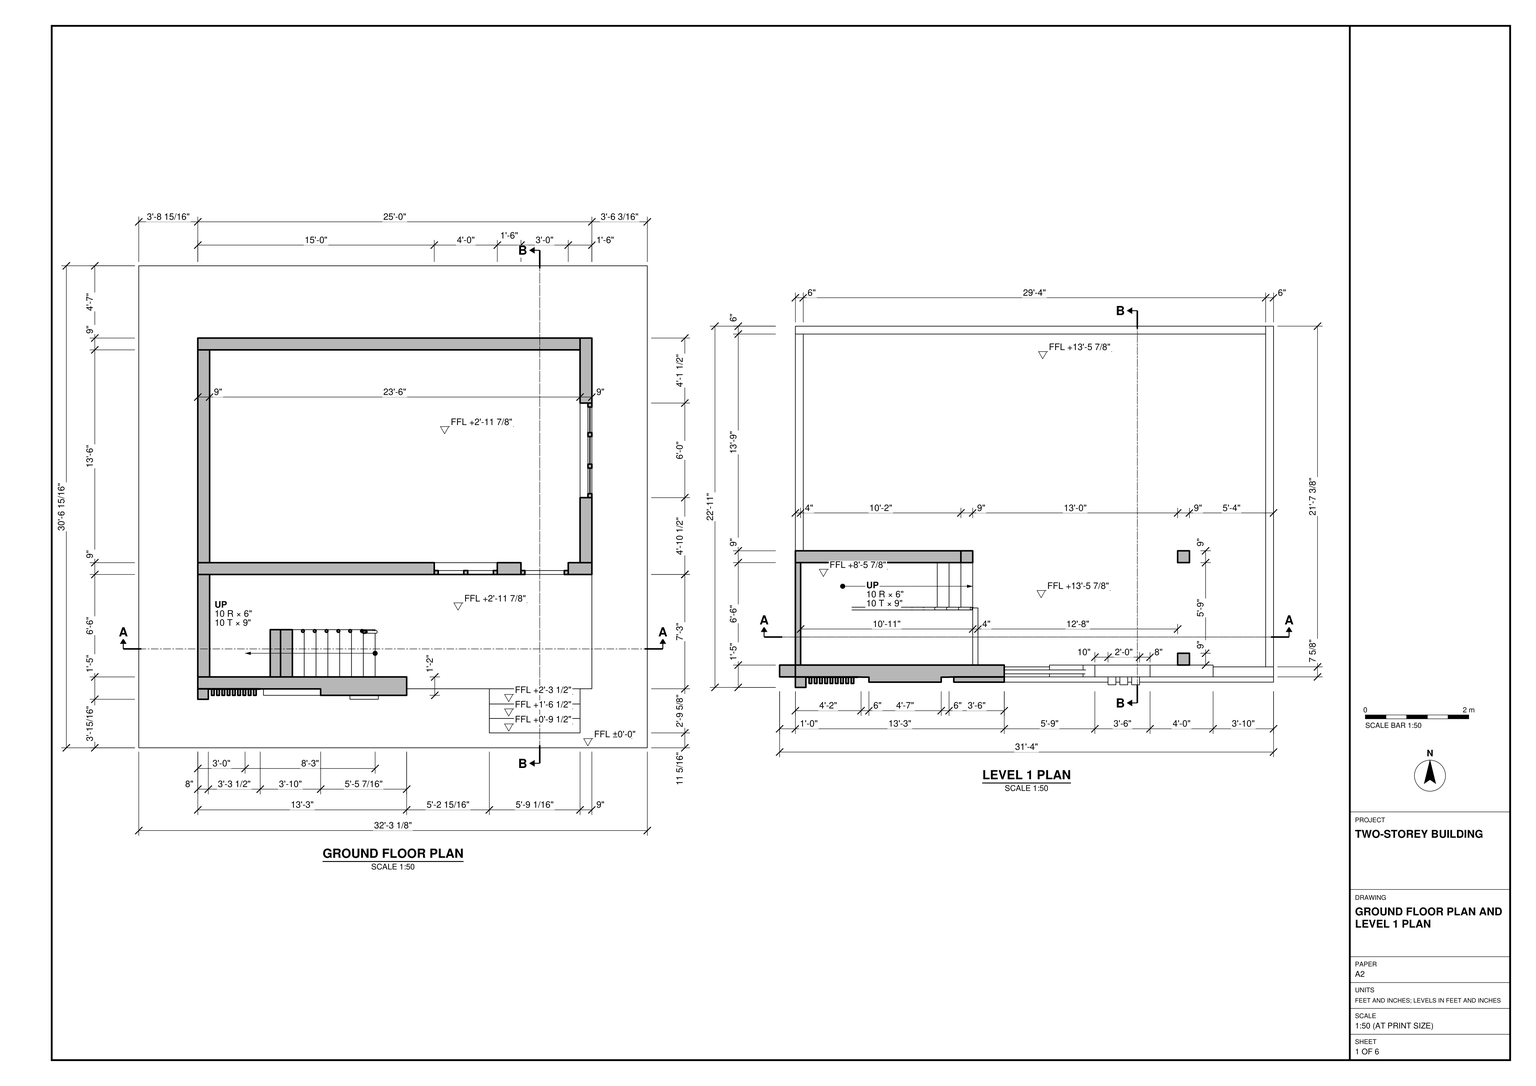
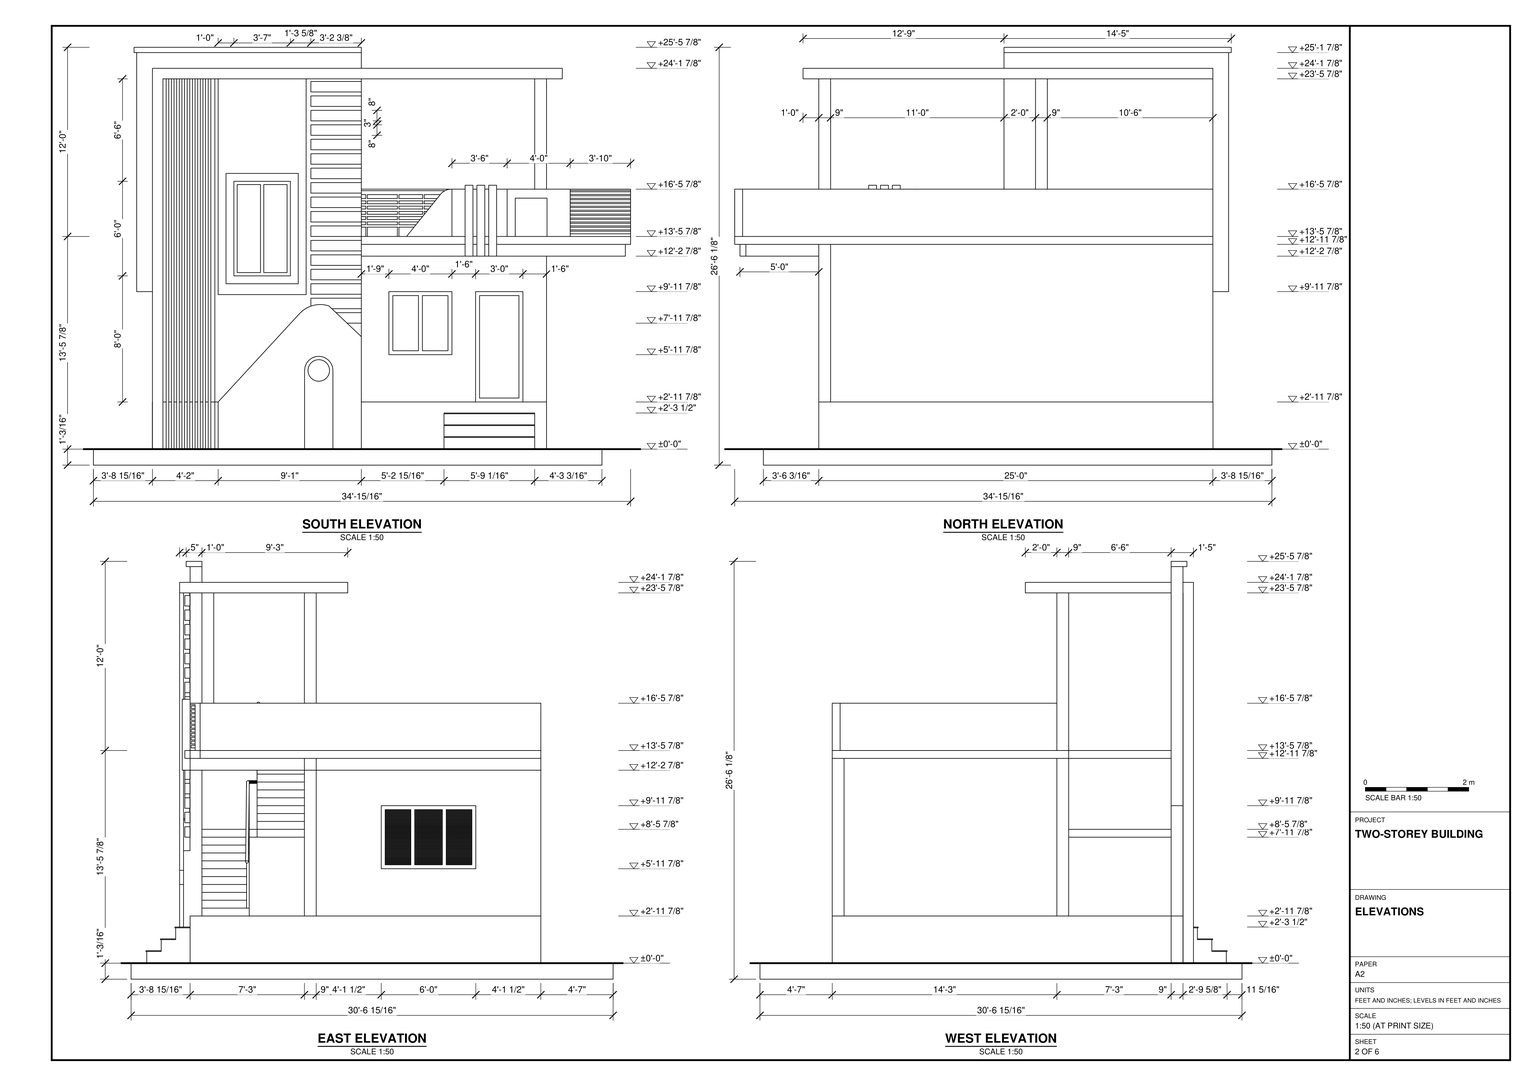
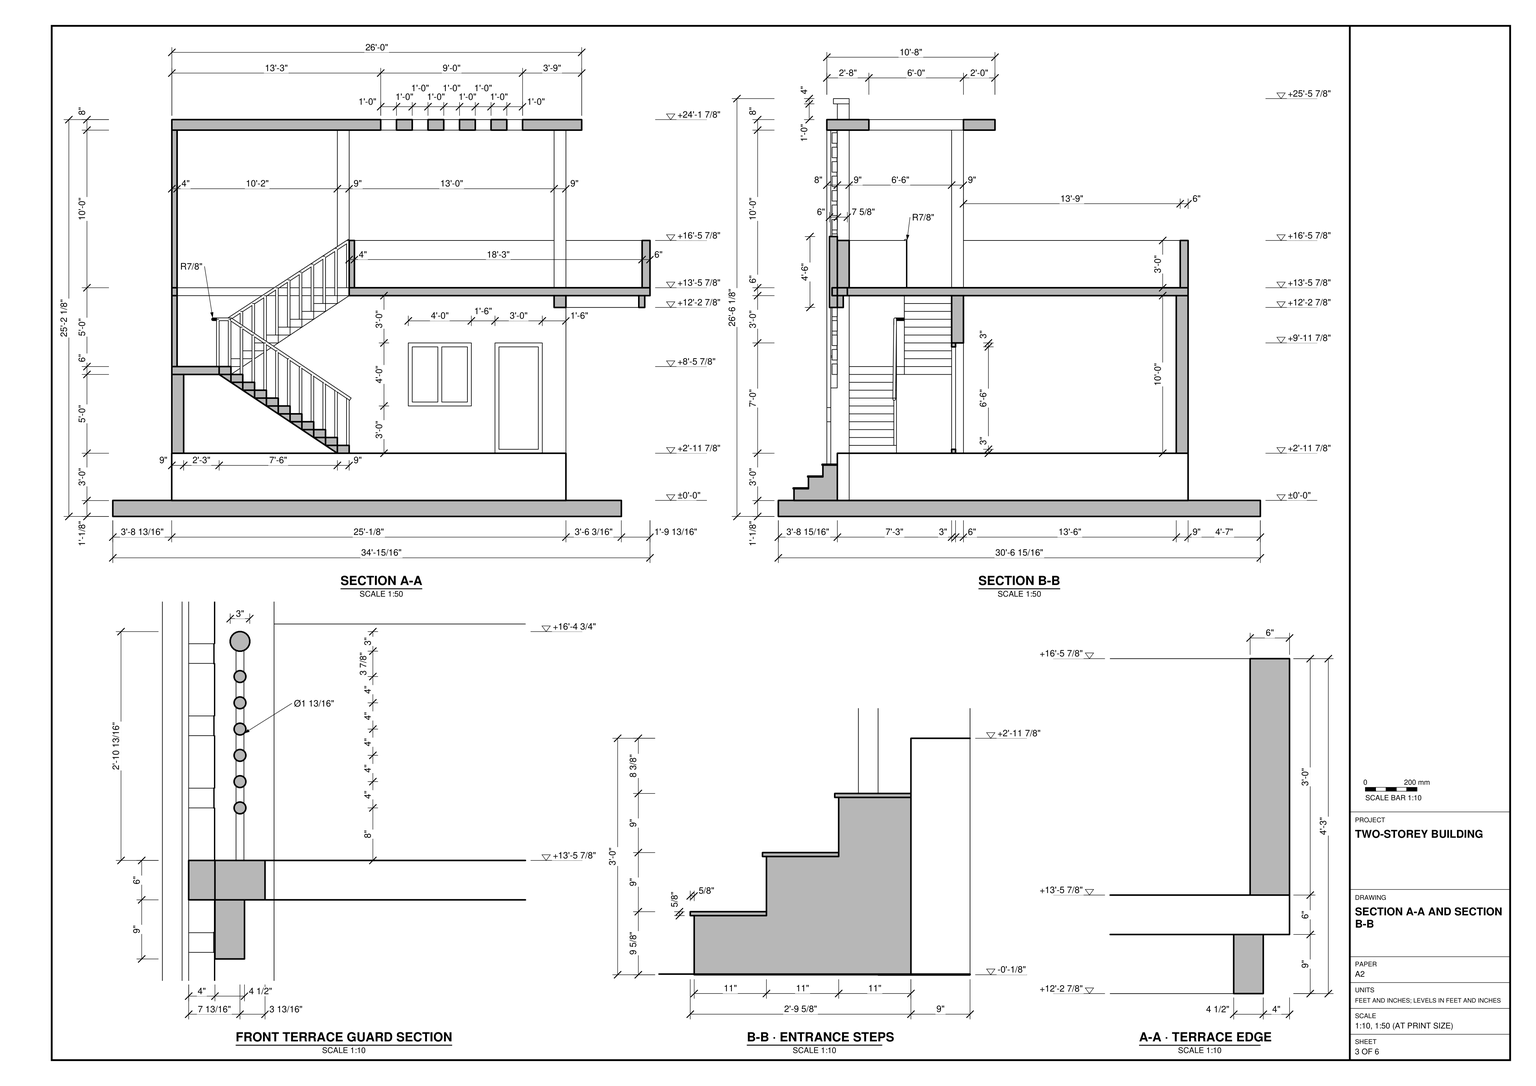
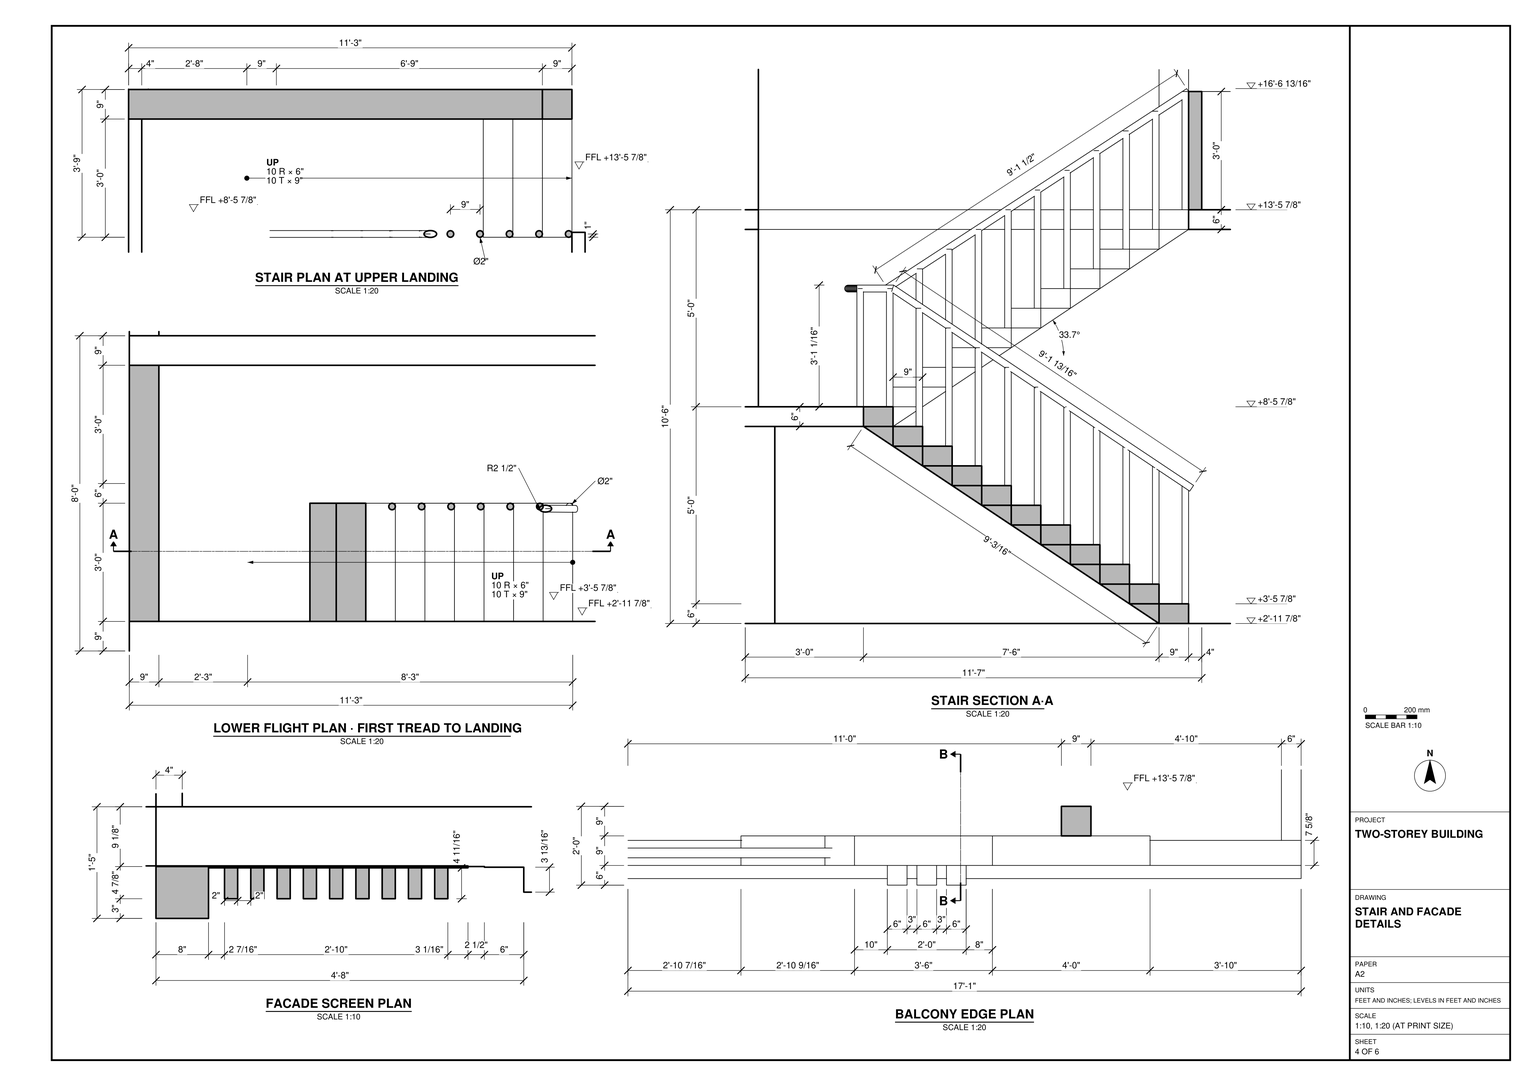
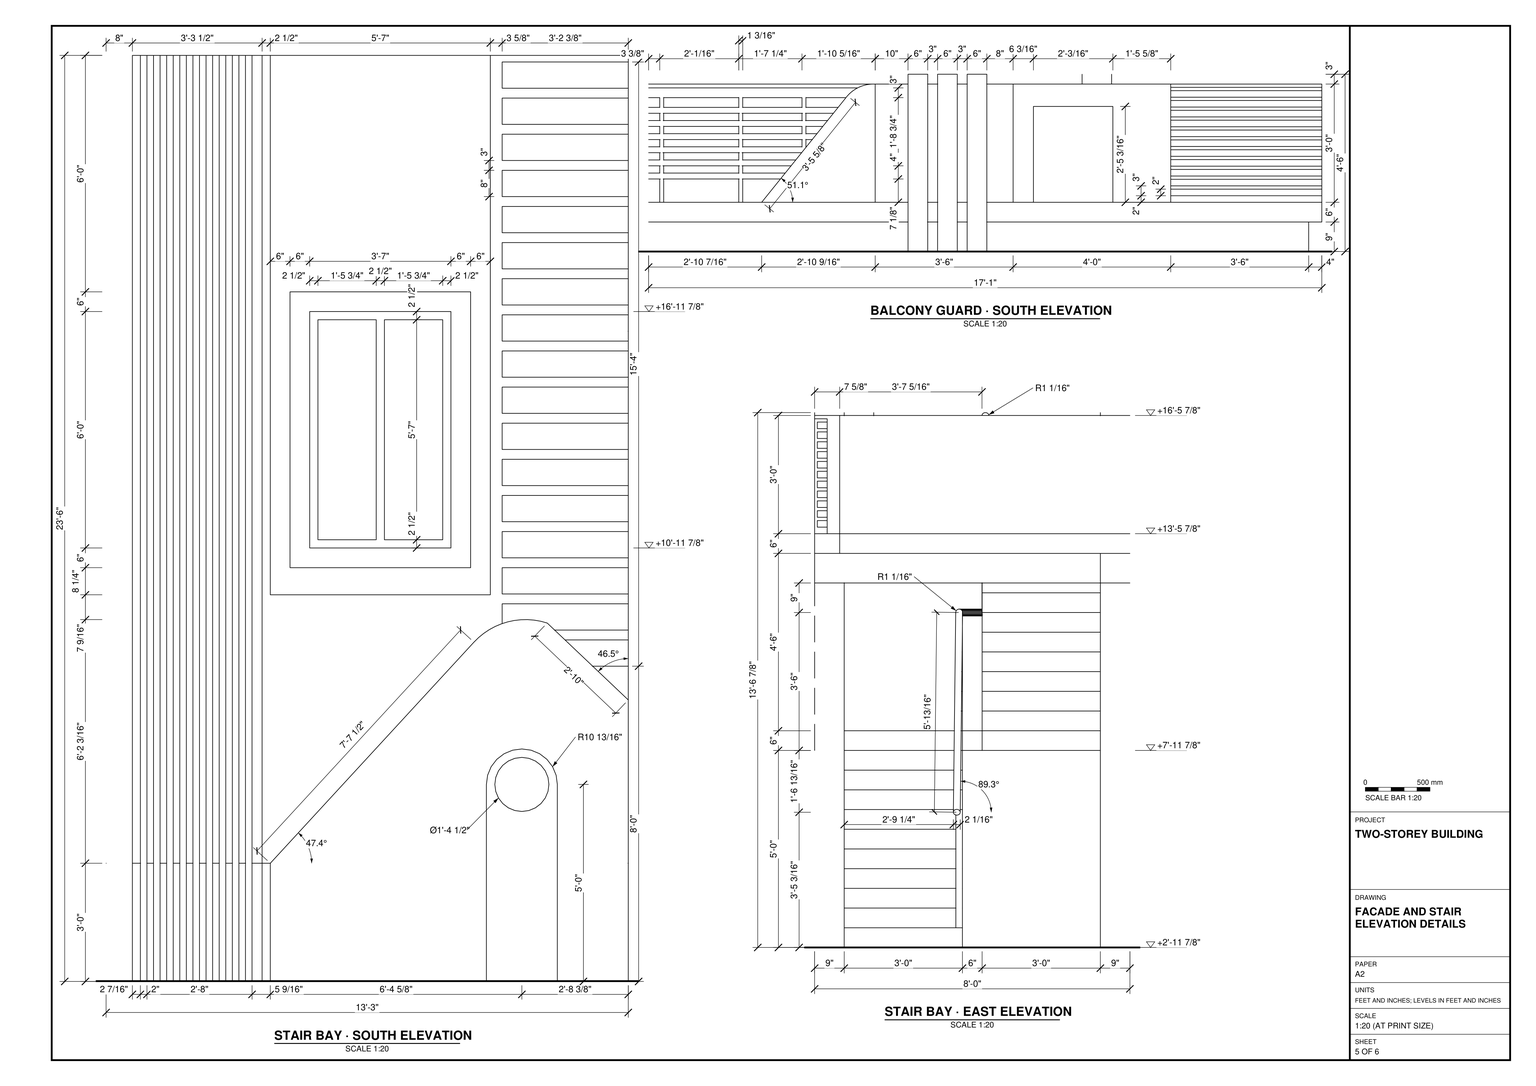
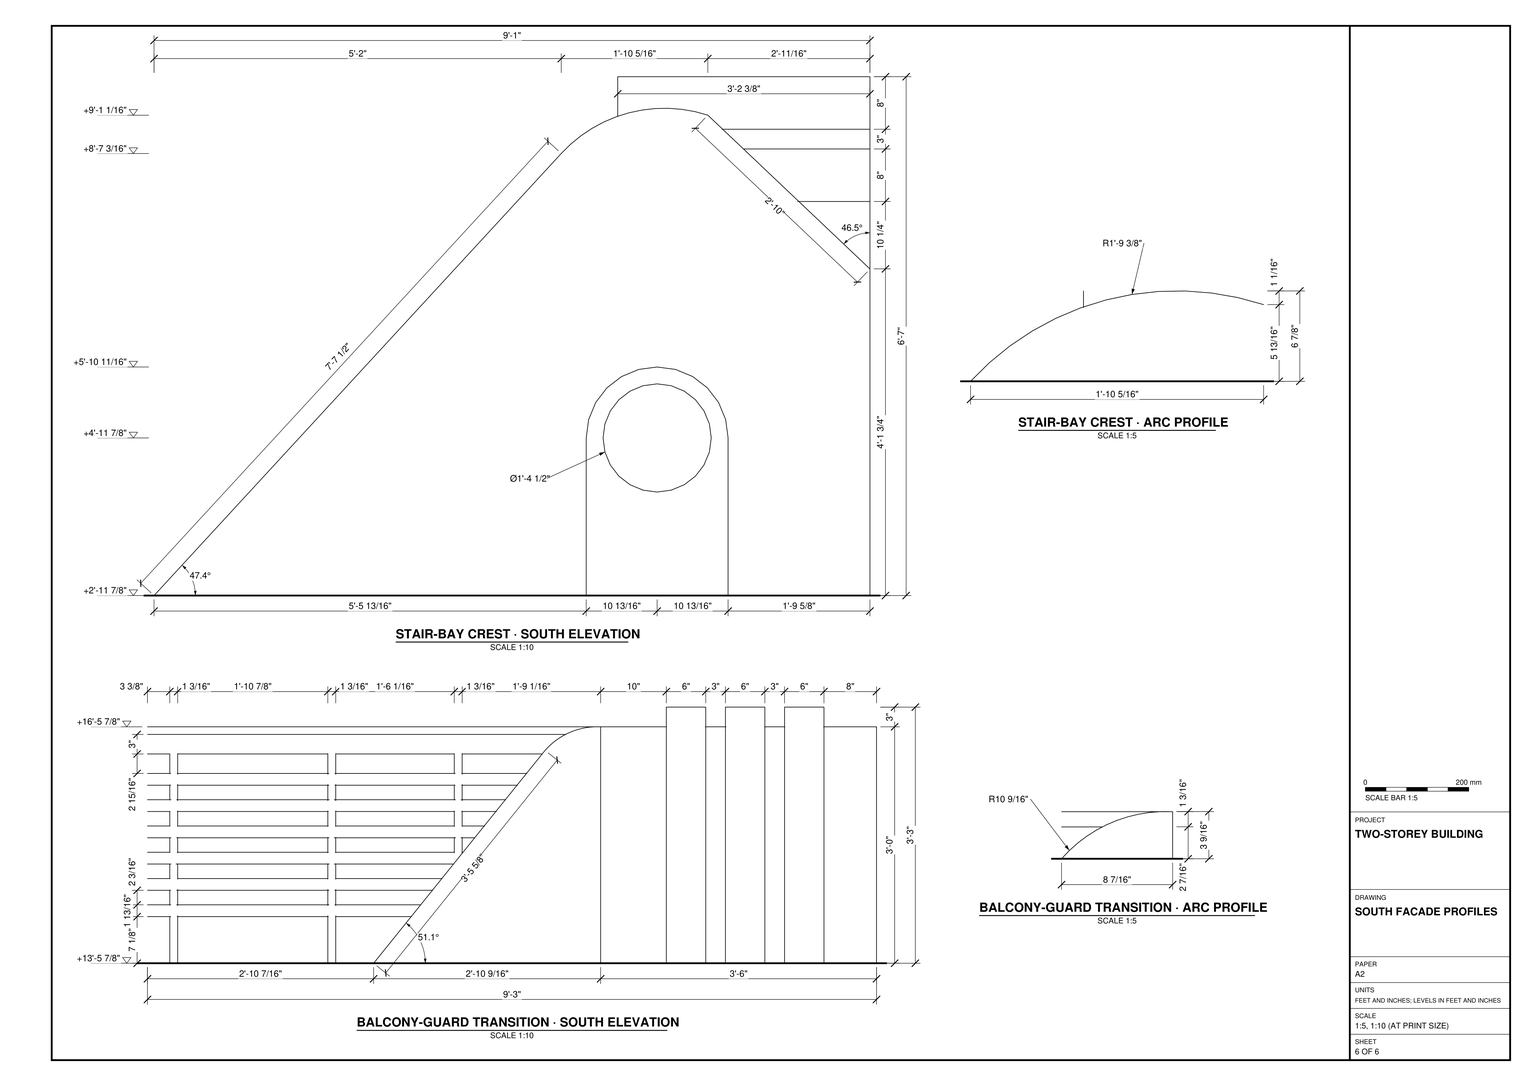
Build the two-storey building in SketchUp from task_files/diagram_01.pdf. Work in feet and inches. The overall extents are 34'-15/16" along X, 30'-6 15/16" along Y and 26'-6 1/8" along Z, including the base slab and projections. Use ±0'-0" as the ground datum and +13'-5 7/8" as the upper floor level.

Model the base slab and the raised ground floor at +2'-11 7/8". Follow the plan for the 9" walls around the rear room, the door and window facing the entrance, and the window in the east wall. On the south side, place the short entrance steps on the right and the return stair on the left. Use the sections to set out the stair flights, intermediate landing and handrails.

Extend the upper slab beyond the room to form the terrace. Follow the terrace edge details for the solid parapets and the horizontal rails across the front. Model the tall south stair screen with its vertical fins, framed window and horizontal bands. Place the partial flat roof on its supports as drawn, leaving the rear terrace open above.

Keep walls, slabs, stairs and roof separate as groups or components. Do the same for each furniture or joinery piece shown, and use components for repeated parts. Decor and loose items may be any suitable library components. Save one SketchUp model as output_files/two_storey_building_with_a_stair_and_upper_terrace.skp.

# SketchUp Ruby script. Lengths in inches.
U = 1.inch
M = Sketchup.active_model
def pt(a) = Geom::Point3d.new(a.map { |v| v * U })
def face(e, loops, mat)
  f = e.add_face(loops[0].map { |a| pt(a) })
  loops[1..].each { |l| e.add_face(l.map { |a| pt(a) }).erase! }
  f.material = f.back_material = mat if mat
  f
end
# faces: each face lists its corners as indices into pts; further lists are holes
def faces(e, pts, list, mat = nil) = list.each { |f| face(e, (f[0].is_a?(Array) ? f : [f]).map { |l| l.map { |i| pts[i] } }, mat) }
# xy, xz, yz: faces in a plane at the given z, y or x. An outline is a flat list of corners, or four numbers for a rectangle; further outlines are holes
def ring(l) = l.size == 4 ? [[l[0], l[1]], [l[2], l[1]], [l[2], l[3]], [l[0], l[3]]] : l.each_slice(2).to_a
def flat(e, list, mat, &to3) = list.each { |f| face(e, (f[0].is_a?(Array) ? f : [f]).map { |l| ring(l).map { |u, v| to3.(u, v) } }, mat) }
def xy(e, z, list, mat = nil) = flat(e, list, mat) { |x, y| [x, y, z] }
def xz(e, y, list, mat = nil) = flat(e, list, mat) { |x, z| [x, y, z] }
def yz(e, x, list, mat = nil) = flat(e, list, mat) { |y, z| [x, y, z] }
def lines(e, pts, list) = list.each { |a, b| e.add_line(pt(pts[a]), pt(pts[b])) }
# prism: a flat outline (further loops are holes) pulled along v
def prism(e, loops, v, mat = nil)
  f = face(e, loops, mat); d = Geom::Vector3d.new(v.map { |x| x * U })
  f.pushpull(f.normal.samedirection?(d) ? d.length : -d.length)
end
def box(e, o, s, mat = nil) = prism(e, [[o, [o[0] + s[0], o[1], o[2]], [o[0] + s[0], o[1] + s[1], o[2]], [o[0], o[1] + s[1], o[2]]]], [0, 0, s[2]], mat)
def at(x, y, z, deg = 0) = Geom::Transformation.translation(pt([x, y, z])) * Geom::Transformation.rotation(ORIGIN, Z_AXIS, deg.degrees)
def axes(o, x, y, z) = Geom::Transformation.new([*x, 0, *y, 0, *z, 0, *pt(o).to_a, 1])
def part(name) = M.definitions.add(name)
# library, detail: a bought-in or finely detailed component or shape, given as its bounding box
def library(name, o, s) = part(name).tap { |d| box(d.entities, o, s) }
def detail(e, o, s) = box(e.add_group.entities, o, s)
def put(e, d, t, mat = nil) = e.add_instance(d, t).tap { |i| i.material = mat if mat }
def group(e, t, mat = nil) = e.add_group.tap { |g| g.transformation = t; g.material = mat if mat }.entities
root = M.entities
M.materials.add("[Aluminum]").color = [179, 179, 179]
M.materials.add("[Color B01]").color = [255, 216, 204]
M.materials.add("[Color B04]").color = [255, 101, 50]
M.materials.add("[Color D07]").color = [153, 114, 0]
M.materials.add("[Color M00]").color = [255, 255, 255]
M.materials.add("[Color M04]").color = [142, 142, 142]
M.materials.add("[Color M05]").color = [114, 114, 114]
M.materials.add("[Color M06]").color = [86, 86, 86]
M.materials.add("[Color M08]").color = [30, 30, 30]
M.materials.add("[Color M09]").color = [0, 0, 0]
M.materials.add("[Metal Corrugated Shiny]").color = [193, 193, 193]
M.materials.add("[Tile Mosaic Multi]").color = [135, 103, 96]
M.materials.add("[Translucent Glass Gray]").color = [128, 128, 128]
M.materials["[Translucent Glass Gray]"].alpha = 0.5
M.materials.add("[Wood Bamboo]").color = [177, 105, 43]
M.materials.add("[Wood Veneer 01]").color = [120, 70, 37]
M.materials.add("[Wood Veneer 02]").color = [190, 128, 91]
c1 = part("Group\#9")
prism(c1.entities,[[[0.01,0,0.22],[0.04,0,0.15],[0.09,0,0.09],[0.15,0,0.04],[0.22,0,0.01],[0.3,0,0],[0.38,0,0.01],[0.45,0,0.04],[0.51,0,0.09],[0.56,0,0.15],[0.59,0,0.22],[0.6,0,0.3],[0.59,0,0.38],[0.56,0,0.45],[0.51,0,0.51],[0.45,0,0.56],[0.38,0,0.59],[0.3,0,0.6],[0.22,0,0.59],[0.15,0,0.56],[0.09,0,0.51],[0.04,0,0.45],[0.01,0,0.38],[0,0,0.3]]],[0,66,0])
c2 = part("Group\#13")
box(c2.entities,[0,0,0],[9,9,120])
c3 = library("Group\#24",[0,0,0],[136.51,78,162.88])
c4 = library("Group\#37",[0,0,0],[69,2.97,34.84])
c5 = part("Group\#40")
box(c5.entities,[0,0,0],[46,3,2])
c6 = part("Group\#50")
box(c6.entities,[0,0,0],[38.4,4,8])
c7 = part("Group\#51")
box(c7.entities,[0,0,0],[2,5,282])
box(root,[0,0,-12.1],[387.125,366.9375,12.2])
xz(root,131.93,[[227.93,75,247.43,117],[250.43,75,269.93,117]],"[Translucent Glass Gray]")
p = [[344.93,44.93,36],[344.93,44.93,27]]
lines(root,p,[[0,1]])
g1 = group(root,at(335.93,53.93,147),"[Color B01]")
box(g1,[0,-4.5,0],[9,82.5,9])
g2 = group(root,at(290.93,131.93,36),"[Wood Bamboo]")
prism(g2,[[[36,3,84],[36,3,0],[0,3,0],[0,3,84]],[[33,3,3],[33,3,81],[3,3,81],[3,3,3]]],[0,-3,0])
g3 = group(root,at(344.93,131.93,147),"[Color M00]")
box(g3,[0,0,0],[60,9,9])
g4 = group(root,at(44.93,131.93,36),"[Color M00]")
prism(g4,[[[300,9,0],[282,9,0],[282,9,84],[246,9,84],[246,9,0],[0,9,0],[0,9,120],[300,9,120]],[[180,9,84],[180,9,36],[228,9,36],[228,9,84]]],[0,-9,0])
g5 = group(root,at(44.93,131.93,0),"[Color M04]")
box(g5,[-0.1,-87,0],[300.1,267,36])
g6 = group(root,at(224.93,131.93,72),"[Color M09]")
prism(g6,[[[0,3,48],[48,3,48],[48,3,0],[0,3,0]],[[3,3,3],[22.5,3,3],[22.5,3,45],[3,3,45]],[[45,3,45],[25.5,3,45],[25.5,3,3],[45,3,3]]],[0,-3,0])
g7 = group(root,at(335.93,140.93,36),"[Color M00]")
prism(g7,[[[9,0,0],[9,171,0],[9,171,120],[9,0,120]],[[9,49.5,84],[9,121.5,84],[9,121.5,36],[9,49.5,36]]],[-9,0,0])
g8 = group(root,at(341.93,190.43,72),"[Color M08]")
put(g8,c1,at(1.2,3,39.35),"[Metal Corrugated Shiny]")
put(g8,c1,at(1.2,3,34.35),"[Metal Corrugated Shiny]")
put(g8,c1,at(1.2,3,36.35),"[Metal Corrugated Shiny]")
put(g8,c1,at(1.2,3,31.35),"[Metal Corrugated Shiny]")
put(g8,c1,at(1.2,3,27.35),"[Metal Corrugated Shiny]")
put(g8,c1,at(1.2,3,28.35),"[Metal Corrugated Shiny]")
put(g8,c1,at(1.2,3,25.35),"[Metal Corrugated Shiny]")
put(g8,c1,at(1.2,3,14.35),"[Metal Corrugated Shiny]")
put(g8,c1,at(1.2,3,44.35),"[Metal Corrugated Shiny]")
put(g8,c1,at(1.2,3,32.35),"[Metal Corrugated Shiny]")
put(g8,c1,at(1.2,3,30.35),"[Metal Corrugated Shiny]")
put(g8,c1,at(1.2,3,26.35),"[Metal Corrugated Shiny]")
put(g8,c1,at(1.2,3,24.35),"[Metal Corrugated Shiny]")
put(g8,c1,at(1.2,3,15.35),"[Metal Corrugated Shiny]")
put(g8,c1,at(1.2,3,29.35),"[Metal Corrugated Shiny]")
put(g8,c1,at(1.2,3,20.35),"[Metal Corrugated Shiny]")
put(g8,c1,at(1.2,3,17.35),"[Metal Corrugated Shiny]")
put(g8,c1,at(1.2,3,16.35),"[Metal Corrugated Shiny]")
put(g8,c1,at(1.2,3,22.35),"[Metal Corrugated Shiny]")
put(g8,c1,at(1.2,3,11.35),"[Metal Corrugated Shiny]")
put(g8,c1,at(1.2,3,10.35),"[Metal Corrugated Shiny]")
put(g8,c1,at(1.2,3,42.35),"[Metal Corrugated Shiny]")
put(g8,c1,at(1.2,3,41.35),"[Metal Corrugated Shiny]")
put(g8,c1,at(1.2,3,38.35),"[Metal Corrugated Shiny]")
put(g8,c1,at(1.2,3,8.35),"[Metal Corrugated Shiny]")
put(g8,c1,at(1.2,3,9.35),"[Metal Corrugated Shiny]")
put(g8,c1,at(1.2,3,21.35),"[Metal Corrugated Shiny]")
put(g8,c1,at(1.2,3,43.35),"[Metal Corrugated Shiny]")
put(g8,c1,at(1.2,3,33.35),"[Metal Corrugated Shiny]")
put(g8,c1,at(1.2,3,23.35),"[Metal Corrugated Shiny]")
g9 = group(g8,at(0,0,0))
prism(g9,[[[3,0,0],[3,72,0],[3,72,48],[3,0,48]],[[3,25.5,45],[3,46.5,45],[3,46.5,3],[3,25.5,3]],[[3,22.5,3],[3,3,3],[3,3,45],[3,22.5,45]],[[3,49.5,45],[3,69,45],[3,69,3],[3,49.5,3]]],[-3,0,0])
put(g8,c1,at(1.2,3,19.35),"[Metal Corrugated Shiny]")
put(g8,c1,at(1.2,3,13.35),"[Metal Corrugated Shiny]")
put(g8,c1,at(1.2,3,12.35),"[Metal Corrugated Shiny]")
put(g8,c1,at(1.2,3,3.35),"[Metal Corrugated Shiny]")
put(g8,c1,at(1.2,3,40.35),"[Metal Corrugated Shiny]")
put(g8,c1,at(1.2,3,35.35),"[Metal Corrugated Shiny]")
put(g8,c1,at(1.2,3,37.35),"[Metal Corrugated Shiny]")
put(g8,c1,at(1.2,3,18.35),"[Metal Corrugated Shiny]")
put(g8,c1,at(1.2,3,6.35),"[Metal Corrugated Shiny]")
put(g8,c1,at(1.2,3,5.35),"[Metal Corrugated Shiny]")
put(g8,c1,at(1.2,3,7.35),"[Metal Corrugated Shiny]")
put(g8,c1,at(1.2,3,4.35),"[Metal Corrugated Shiny]")
g10 = group(root,at(44.93,140.93,36),"[Color M00]")
xy(g10,0,[[0,0,9,162],[0,162,291,171]])
xy(g10,120,[[0,0,9,162],[0,162,291,171]])
xz(g10,0,[[0,0,9,120]])
xz(g10,162,[[0,0,9,120],[9,0,291,120]])
xz(g10,171,[[0,0,291,120]])
yz(g10,0,[[0,0,162,120],[162,0,171,120]])
yz(g10,9,[[0,0,162,120]])
yz(g10,291,[[162,0,171,120]])
g11 = group(root,at(44.93,53.93,156),"[Color M00]")
xy(g11,0,[[159,-13,364,-9],[159,-9,364,-1.375],[159,-1.375,159,0,135,0,135,78,4,78,4,0,0,0,0,258,364,258,364,-1.375]],"[Color M00]")
xy(g11,6,[[159,-9,364,-1.375],[159,-1.375,364,-1.375,364,258,0,258,0,0,4,0,4,78,135,78,135,0,159,0]],"[Color M00]")
xy(g11,6,[[159,-13,364,-9]],"[Wood Veneer 01]")
xz(g11,-13,[[159,0,364,6]],"[Wood Veneer 01]")
xz(g11,-9,[[159,0,364,6]],"[Color M00]")
xz(g11,-1.375,[[159,0,364,6]],"[Color M00]")
xz(g11,0,[[0,0,4,6],[135,0,159,6]],"[Color M00]")
xz(g11,78,[[4,0,135,6]],"[Color M00]")
xz(g11,258,[[0,0,364,6]],"[Color M00]")
yz(g11,0,[[0,0,78,6],[78,0,258,6]],"[Color M00]")
yz(g11,4,[[0,0,78,6]],"[Color M00]")
yz(g11,135,[[0,0,78,6]],"[Color M00]")
yz(g11,159,[[-13,0,-9,6],[-9,0,-1.375,6],[-1.375,0,0,6]],"[Color M00]")
yz(g11,364,[[-9,0,-1.375,6],[-1.375,0,258,6]],"[Color M00]")
yz(g11,364,[[-13,0,-9,6]],"[Wood Veneer 01]")
put(root,c2,at(335.93,131.93,162),"[Color M00]")
g12 = group(root,at(44.93,53.93,102),"[Color M00]")
box(g12,[0,0,0],[4,78,54])
put(root,c3,at(44.93,53.93,36),"[Color M00]")
put(root,c2,at(170.93,131.93,162),"[Color M00]")
g13 = group(root,at(44.93,131.93,162),"[Color M00]")
box(g13,[0,0,0],[126,9,120])
g14 = group(root,at(44.93,53.93,162),"[Color M00]")
box(g14,[0,0,0],[4,78,120])
g15 = group(root,at(44.93,44.93,36),"[Color M00]")
xy(g15,-36.1,[[50,-5,50,-0.1,0,-0.1,0,9,159,9,159,-5]])
xy(g15,81.74,[[50,-0.2,117,-0.1]])
xy(g15,90,[[56,-4,111,-0.2]])
xy(g15,96,[[62,-4,105,9]])
xy(g15,168,[[62,-4,105,9]])
xy(g15,174,[[56,-4,111,-0.2]])
xy(g15,246,[[50,-0.2,117,-0.2,117,-0.1,159,-0.1,159,9,0,9,0,-0.1,50,-0.1]])
xz(g15,-4,[[[56,90,111,174],[62,96,105,168]]])
xz(g15,-0.1,[[0,-36.1,50,-36.1,50,0,112,67.3125,113.44,68.74,115.02,70.02,116.71,71.15,118.49,72.11,120.36,72.9,122.3,73.5,124.29,73.92,126.3,74.15,128.33,74.19,130.36,74.03,132.35,73.6875,134.3125,73.15,159,49.73,159,246,117,246,117,81.74,50,81.74,50,246,0,246]])
xz(g15,9,[[[0,-36.1,159,246],[62,96,105,168]]])
yz(g15,0,[[-0.1,-36.1,9,246]])
yz(g15,50,[[-5,-36.1,-0.1,0],[-0.2,81.74,-0.1,246]])
yz(g15,56,[[-4,90,-0.2,174]])
yz(g15,62,[[-4,96,9,168]])
yz(g15,105,[[-4,96,9,168]])
yz(g15,111,[[-4,90,-0.2,174]])
yz(g15,117,[[-0.2,81.74,-0.1,246]])
yz(g15,159,[[-5,-36.1,9,-36.1,9,246,-0.1,246,-0.1,49.73,-5,49.73]])
p = [[112,-0.1,67.3125],[50,-0.1,0],[50,-5,0],[112,-5,67.3125],[159,-0.1,49.73],[134.3125,-0.1,73.15],
  [134.3125,-5,73.15],[159,-5,49.73],[113.44,-0.1,68.74],[113.44,-5,68.74],[115.02,-0.1,70.02],[115.02,-5,70.02],
  [116.71,-0.1,71.15],[116.71,-5,71.15],[118.49,-0.1,72.11],[118.49,-5,72.11],[120.36,-0.1,72.9],[120.36,-5,72.9],
  [122.3,-0.1,73.5],[122.3,-5,73.5],[132.35,-0.1,73.6875],[132.35,-5,73.6875],[124.29,-0.1,73.92],[124.29,-5,73.92],
  [130.36,-0.1,74.03],[130.36,-5,74.03],[126.3,-0.1,74.15],[126.3,-5,74.15],[128.33,-0.1,74.19],[128.33,-5,74.19]]
faces(g15,p,[[0,1,2,3],[4,5,6,7],[8,0,3,9],[10,8,9,11],[12,10,11,13],[14,12,13,15],[16,14,15,17],[18,16,17,19],
  [5,20,21,6],[22,18,19,23],[20,24,25,21],[26,22,23,27],[24,28,29,25],[28,26,27,29]])
g16 = group(g15,at(50,-0.2,81.74))
xz(g16,0,[[[0,0,67,164.26],[6,8.26,61,92.26]]],"[Color M06]")
g17 = group(g15,at(50,-5,-36))
xz(g17,0,[[0,0,109,0,109,85.73,84.3125,109.15,82.35,109.6875,80.36,110.03,78.33,110.19,76.3,110.15,74.29,109.92,72.3,109.5,70.36,108.9,68.49,108.11,66.71,107.15,65.02,106.02,63.44,104.74,62,103.3125,0,36]],"[Color D07]")
put(root,c2,at(335.93,53.93,162),"[Color M00]")
g18 = group(root,at(44.93,44.93,282),"[Wood Veneer 01]")
xy(g18,-282,[[0,-8,8,0]])
xy(g18,0,[[[8,-8,8,0,0,0,0,120,312,120,312,-8],[183,24,195,96],[207,24,219,96],[231,24,243,96],[255,24,267,96],[159,24,171,96]]])
xy(g18,8,[[[0,-8,312,120],[183,24,195,96],[207,24,219,96],[231,24,243,96],[255,24,267,96],[159,24,171,96]]])
xz(g18,-8,[[0,-282,8,-282,8,0,312,0,312,8,0,8]])
xz(g18,0,[[0,-282,8,0]])
xz(g18,24,[[159,0,171,8],[183,0,195,8],[207,0,219,8],[231,0,243,8],[255,0,267,8]])
xz(g18,96,[[159,0,171,8],[183,0,195,8],[207,0,219,8],[231,0,243,8],[255,0,267,8]])
xz(g18,120,[[0,0,312,8]])
yz(g18,0,[[-8,-282,-8,8,120,8,120,0,0,0,0,-282]])
yz(g18,8,[[-8,-282,0,0]])
yz(g18,159,[[24,0,96,8]])
yz(g18,171,[[24,0,96,8]])
yz(g18,183,[[24,0,96,8]])
yz(g18,195,[[24,0,96,8]])
yz(g18,207,[[24,0,96,8]])
yz(g18,219,[[24,0,96,8]])
yz(g18,231,[[24,0,96,8]])
yz(g18,243,[[24,0,96,8]])
yz(g18,255,[[24,0,96,8]])
yz(g18,267,[[24,0,96,8]])
yz(g18,312,[[-8,0,120,8]])
g19 = group(root,at(44.93,53.93,36),"[Color M00]")
box(g19,[0,0,0],[9,78,60])
g20 = group(root,at(179.93,53.93,162),"[Color M00]")
box(g20,[0,0,0],[4,43.5,36])
g21 = group(root,at(203.93,44.93,147),"[Color M00]")
prism(g21,[[[201,0,0],[0,0,0],[0,4.5,0],[196.5,4.5,0],[196.5,267,0],[201,267,0]]],[0,0,9])
g22 = group(root,at(272.93,44.93,162),"[Color M06]")
box(g22,[0,0,0],[42,9,36])
g23 = group(root,at(314.93,44.93,162),"[Color D07]")
xy(g23,0,[[0,0,0,9,48,9,48,0,30.375,0,30.375,7.625,6.1875,7.625,6.1875,0]])
xy(g23,29.1875,[[6.1875,0,30.375,7.625]])
xy(g23,36,[[0,0,48,9]])
xz(g23,0,[[0,0,6.1875,0,6.1875,29.1875,30.375,29.1875,30.375,0,48,0,48,36,0,36]])
xz(g23,7.625,[[6.1875,0,30.375,29.1875]],"[Color M00]")
xz(g23,9,[[0,0,48,36]])
yz(g23,0,[[0,0,9,36]])
yz(g23,6.1875,[[0,0,7.625,29.1875]])
yz(g23,30.375,[[0,0,7.625,29.1875]])
yz(g23,48,[[0,0,9,36]])
g24 = group(root,at(238.36,44.93,162),"[Color M05]")
prism(g24,[[[34.57,9,0],[0,9,0],[25.57,9,31.74],[26.11,9,32.42],[26.71,9,33.04],[27.35,9,33.62],[28.04,9,34.14],[28.77,9,34.6],[29.54,9,35],[30.33,9,35.34],[31.15,9,35.61],[31.99,9,35.8125],[32.84,9,35.95],[33.71,9,36.01],[34.57,9,36]]],[0,-9,0])
put(root,c4,at(203.93,47.25,162),"[Aluminum]")
g25 = group(root,at(282.93,40.93,162),"[Color M00]")
box(g25,[9,-2,-15],[6,6,54])
box(g25,[18,-2,-15],[6,6,54])
box(g25,[0,-2,-15],[6,6,54])
g26 = group(root,at(362.93,44.93,162),"[Color B04]")
put(g26,c5,at(0,0.8125,32))
put(g26,c5,at(0,0.8125,23))
put(g26,c5,at(0,0.8125,8))
put(g26,c5,at(0,0.8125,14))
put(g26,c5,at(0,0.8125,2))
put(g26,c5,at(0,0.8125,5))
g27 = group(g26,at(0,0,0))
prism(g27,[[[0,7.625,0],[0,3.8125,0],[0,3.8125,35],[0,0,35],[0,0,36],[0,7.625,36]]],[46,0,0])
put(g26,c5,at(0,0.8125,20))
put(g26,c5,at(0,0.8125,17))
put(g26,c5,at(0,0.8125,11))
put(g26,c5,at(0,0.8125,26))
put(g26,c5,at(0,0.8125,29))
g28 = group(root,at(402.93,52.55,162),"[Color M00]")
box(g28,[0,0,0],[6,259.375,36])
g29 = group(root,at(44.93,305.93,162),"[Color M00]")
box(g29,[0,0,0],[358,6,36])
g30 = group(root,at(44.93,140.93,162),"[Color M00]")
box(g30,[0,0,0],[6,165,36])
g31 = group(root,at(32.93,44.93,120),"[Color M00]")
prism(g31,[[[12,0,170],[171,0,170],[171,0,182],[0,0,182],[0,0,0],[12,0,0]]],[0,9,0])
g32 = group(root,at(30.93,41.93,302),"[Wood Veneer 01]")
box(g32,[0,0,0],[173,12,4])
g33 = group(root,at(106.93,40.93,132),"[Color M09]")
prism(g33,[[[0,0,72],[0,0,0],[43,0,0],[43,0,72]],[[22.75,0,2.5],[22.75,0,69.5],[40.5,0,69.5],[40.5,0,2.5]],[[20.25,0,2.5],[2.5,0,2.5],[2.5,0,69.5],[20.25,0,69.5]]],[0,3,0])
g34 = group(root,at(109.43,42.43,134.5),"[Translucent Glass Gray]")
xz(g34,0,[[0,0,17.75,67],[20.25,0,38,67]])
g35 = group(root,at(165.53,40.93,96),"[Color B04]")
put(g35,c6,at(0,0,143))
put(g35,c6,at(0,0,88))
put(g35,c6,at(0,0,11))
put(g35,c6,at(0,0,176))
put(g35,c6,at(0,0,154))
put(g35,c6,at(0,0,77))
put(g35,c6,at(0,0,121))
put(g35,c6,at(0,0,99))
put(g35,c6,at(0,0,33))
put(g35,c6,at(0,0,165))
put(g35,c6,at(0,0,66))
put(g35,c6,at(0,0,55))
put(g35,c6,at(0,0,110))
g36 = group(g35,at(0,0,0))
box(g36,[0,0,0],[38.4,4,8])
put(g35,c6,at(0,0,44))
put(g35,c6,at(0,0,132))
put(g35,c6,at(0,0,22))
g37 = group(root,at(160.73,36.93,0),"[Color M00]")
prism(g37,[[[0,0,60],[0,0,0],[21.6,0,0],[21.6,0,60],[21.23,0,62.8],[20.15,0,65.4],[18.4375,0,67.64],[16.2,0,69.35],[13.6,0,70.43],[10.8,0,70.8],[8,0,70.43],[5.4,0,69.35],[3.16,0,67.64],[1.45,0,65.4],[0.37,0,62.8]],[[16.62,0,54.18],[14.92,0,52.87],[12.93,0,52.05],[10.8,0,51.77],[8.67,0,52.05],[6.68,0,52.87],[4.98,0,54.18],[3.67,0,55.88],[2.85,0,57.87],[2.57,0,60],[2.85,0,62.13],[3.67,0,64.12],[4.98,0,65.82],[6.68,0,67.13],[8.67,0,67.95],[10.8,0,68.23],[12.93,0,67.95],[14.92,0,67.13],[16.62,0,65.82],[17.93,0,64.12],[18.75,0,62.13],[19.03,0,60],[18.75,0,57.87],[17.93,0,55.88]]],[0,3,0])
g38 = group(root,at(55.37,39.93,0))
put(g38,c7,at(32,0,0),"[Wood Veneer 02]")
put(g38,c7,at(28,0,0),"[Wood Veneer 02]")
put(g38,c7,at(4,0,0),"[Wood Veneer 02]")
put(g38,c7,at(8,0,0),"[Wood Veneer 02]")
put(g38,c7,at(16,0,0),"[Wood Veneer 02]")
put(g38,c7,at(20,0,0),"[Wood Veneer 02]")
put(g38,c7,at(0,0,0),"[Wood Veneer 02]")
put(g38,c7,at(12,0,0),"[Wood Veneer 02]")
put(g38,c7,at(24,0,0),"[Wood Veneer 02]")
g39 = group(root,at(52.93,44.63,0),"[Wood Veneer 02]")
box(g39,[0,0,0],[39.5,0.3,282])
g40 = group(root,at(266.87,11.33,0))
xy(g40,9,[[0,0,69.0625,11.6]])
xy(g40,9.6,[[0,0,69.0625,11.6]],"[Tile Mosaic Multi]")
xy(g40,18,[[0,11,69.0625,22.6]])
xy(g40,18.6,[[0,11,69.0625,22.6]],"[Tile Mosaic Multi]")
xy(g40,27,[[0,22,69.0625,33.6]])
xy(g40,27.6,[[0,22,69.0625,33.6]],"[Tile Mosaic Multi]")
xz(g40,0,[[0,9,69.0625,9.6]])
xz(g40,11,[[0,18,69.0625,18.6]])
xz(g40,11.6,[[0,9,69.0625,9.6]])
xz(g40,22,[[0,27,69.0625,27.6]])
xz(g40,22.6,[[0,18,69.0625,18.6]])
xz(g40,33.6,[[0,27,69.0625,27.6]])
yz(g40,0,[[0,9,11.6,9.6],[11,18,22.6,18.6],[22,27,33.6,27.6]])
yz(g40,69.0625,[[0,9,11.6,9.6],[11,18,22.6,18.6],[22,27,33.6,27.6]])
g41 = group(g40,at(-7.1875,0.6,0),"[Color M05]")
g42 = group(g41,at(7.1875,0,0))
prism(g42,[[[69.0625,33,27],[69.0625,33,0],[69.0625,0,0],[69.0625,0,9],[69.0625,11,9],[69.0625,11,18],[69.0625,22,18],[69.0625,22,27]]],[-69.0625,0,0])
